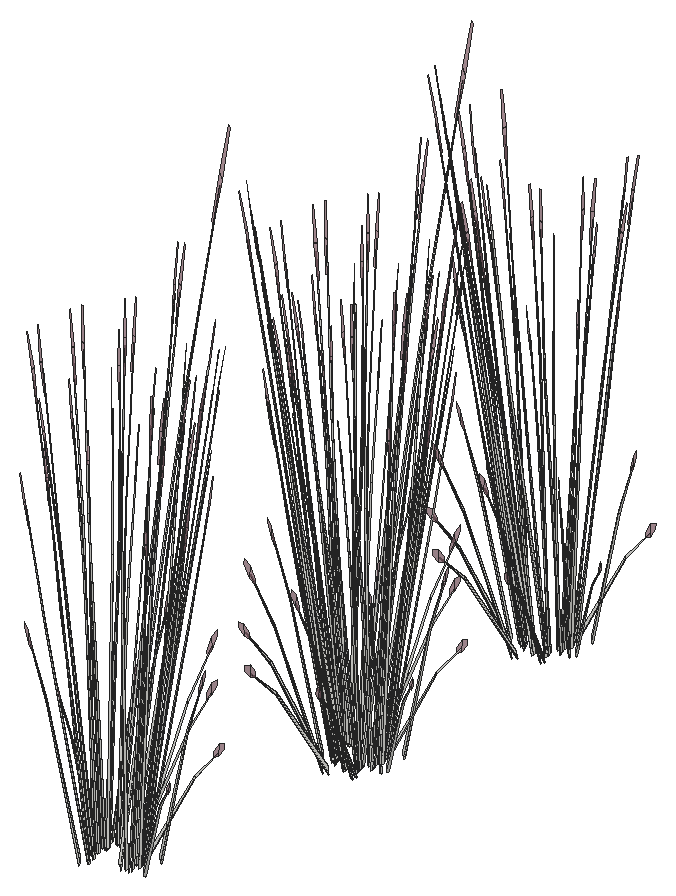
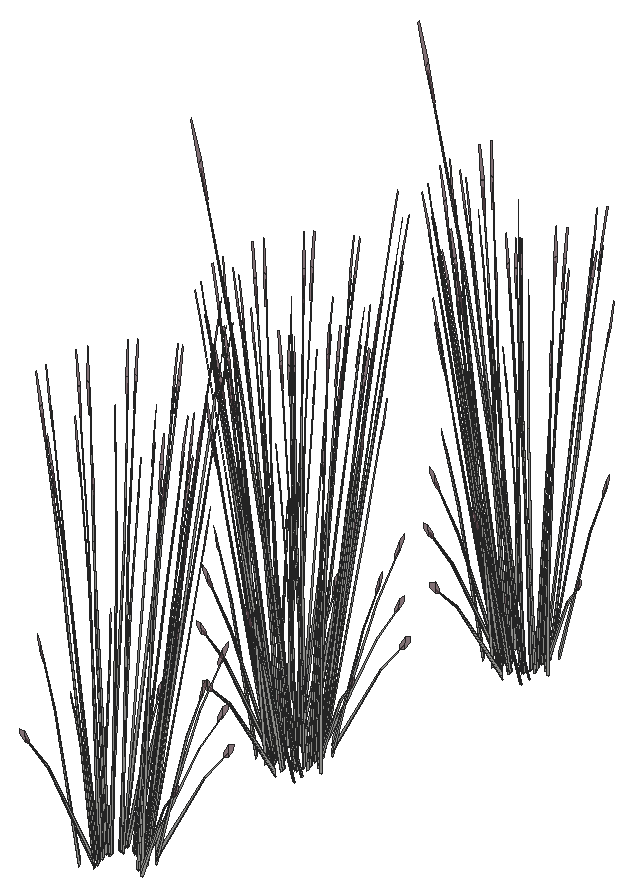
# SketchUp Ruby script. Lengths in inches.
U = 1.inch
M = Sketchup.active_model
def pt(a) = Geom::Point3d.new(a.map { |v| v * U })
def face(e, loops, mat)
  f = e.add_face(loops[0].map { |a| pt(a) })
  loops[1..].each { |l| e.add_face(l.map { |a| pt(a) }).erase! }
  f.material = f.back_material = mat if mat
  f
end
# faces: each face lists its corners as indices into pts; further lists are holes
def faces(e, pts, list, mat = nil) = list.each { |f| face(e, (f[0].is_a?(Array) ? f : [f]).map { |l| l.map { |i| pts[i] } }, mat) }
# xy, xz, yz: faces in a plane at the given z, y or x. An outline is a flat list of corners, or four numbers for a rectangle; further outlines are holes
def ring(l) = l.size == 4 ? [[l[0], l[1]], [l[2], l[1]], [l[2], l[3]], [l[0], l[3]]] : l.each_slice(2).to_a
def flat(e, list, mat, &to3) = list.each { |f| face(e, (f[0].is_a?(Array) ? f : [f]).map { |l| ring(l).map { |u, v| to3.(u, v) } }, mat) }
def xy(e, z, list, mat = nil) = flat(e, list, mat) { |x, y| [x, y, z] }
def xz(e, y, list, mat = nil) = flat(e, list, mat) { |x, z| [x, y, z] }
def yz(e, x, list, mat = nil) = flat(e, list, mat) { |y, z| [x, y, z] }
def lines(e, pts, list) = list.each { |a, b| e.add_line(pt(pts[a]), pt(pts[b])) }
# prism: a flat outline (further loops are holes) pulled along v
def prism(e, loops, v, mat = nil)
  f = face(e, loops, mat); d = Geom::Vector3d.new(v.map { |x| x * U })
  f.pushpull(f.normal.samedirection?(d) ? d.length : -d.length)
end
def box(e, o, s, mat = nil) = prism(e, [[o, [o[0] + s[0], o[1], o[2]], [o[0] + s[0], o[1] + s[1], o[2]], [o[0], o[1] + s[1], o[2]]]], [0, 0, s[2]], mat)
def at(x, y, z, deg = 0) = Geom::Transformation.translation(pt([x, y, z])) * Geom::Transformation.rotation(ORIGIN, Z_AXIS, deg.degrees)
def axes(o, x, y, z) = Geom::Transformation.new([*x, 0, *y, 0, *z, 0, *pt(o).to_a, 1])
def part(name) = M.definitions.add(name)
# library, detail: a bought-in or finely detailed component or shape, given as its bounding box
def library(name, o, s) = part(name).tap { |d| box(d.entities, o, s) }
def detail(e, o, s) = box(e.add_group.entities, o, s)
def put(e, d, t, mat = nil) = e.add_instance(d, t).tap { |i| i.material = mat if mat }
def group(e, t, mat = nil) = e.add_group.tap { |g| g.transformation = t; g.material = mat if mat }.entities
root = M.entities
M.materials.add("LightPink_Translucent").color = [144, 107, 117]
M.materials["LightPink_Translucent"].alpha = 0.75
c1 = part("blade")
p = [[2.15,0.21,22],[0,0.17,0],[0.09,0.45,0],[2.18,0.31,22],[2.29,0.31,22],[0.38,0.45,0],
  [2.48,0.24,33],[2.49,0.24,33],[2.48,0.22,33]]
faces(c1.entities,p,[[0,1,2,3],[4,5,2,3],[6,3,4,7],[8,0,3,6]])
c2 = part("seeds")
p = [[0.3,-0.1,1.38],[-0.01,-0.03,1.59],[-0.01,-0.03,0.03],[0.14,-0.07,-0.07],[0.29,-0.03,3],[0.15,0.01,3.11]]
faces(c2.entities,p,[[0,1,2,3],[1,0,4,5]],"LightPink_Translucent")
c3 = part("blade with seeds")
put(c3.entities,c1,at(0,0,0))
put(c3.entities,c2,axes([2.4,0.25,30.99],[1.5799,-0.05474,1.17369],[-0.12525,1.92788,0.29478],[-0.07173,-0.02425,1.56792]))
put(root,c3,axes([397.1875,39.03,4.73],[0.01777,-0.35463,0.0643],[0.26836,0.00972,0.50621],[-0.1028,-0.03711,0.77189]))
put(root,c3,axes([399.82,39.89,5.05],[-0.30722,0.06665,0.35414],[-0.08112,-0.381,-0.4572],[0.08804,-0.10234,0.87481]))
put(root,c3,axes([400.1,39.83,4.73],[0.2423,0.19613,0.0643],[-0.14107,0.2793,0.50621],[0.07768,-0.0903,0.77189]))
put(root,c3,axes([400.03,39.75,4.73],[0.08753,0.42921,0.48003],[-0.34336,0.07449,0.3958],[0.1012,-0.10094,0.9933]))
put(root,c3,axes([400.96,40.27,4.72],[0.04898,-0.07104,1.74944],[-0.06269,-0.43574,-0.27667],[0.12289,-0.08262,0.14031]))
put(root,c3,axes([396.82,38.57,4.71],[0.02617,0.04654,1.77383],[-0.12614,0.41836,-0.16761],[-0.12775,0.00303,0.31391]))
put(root,c3,axes([397.37,39.3,5.05],[0.20082,0.29199,0.35414],[-0.2293,0.2764,-0.4572],[-0.1165,-0.04206,0.87481]))
put(root,c3,axes([397.32,39.11,5.03],[-0.0189,0.47427,-0.1216],[-0.35781,-0.01296,-0.67495],[-0.13781,-0.03295,1.02557]))
put(root,c3,axes([399.99,40.93,5.03],[-0.17758,-0.42229,-0.1216],[0.31518,-0.20752,-0.67495],[0.13282,-0.05572,1.02557]))
put(root,c3,axes([399.87,40.81,5.05],[-0.29332,-0.1301,0.35414],[0.08555,-0.37955,-0.4572],[0.11809,-0.0348,0.87481]))
put(root,c3,axes([396.8,40.11,4.73],[0.09971,-0.42522,0.48003],[0.32782,0.1454,0.3958],[-0.12892,0.02555,0.9933]))
put(root,c3,axes([396.77,40,4.73],[-0.12963,-0.31798,0.0643],[0.23638,-0.15564,0.50621],[-0.1042,0.03071,0.77189]))
put(root,c3,axes([400.14,40.92,4.73],[0.12963,0.31798,0.0643],[-0.23638,0.15564,0.50621],[0.1042,-0.03071,0.77189]))
put(root,c3,axes([400.11,40.81,4.73],[-0.09971,0.42522,0.48003],[-0.32782,-0.1454,0.3958],[0.12892,-0.02555,0.9933]))
put(root,c3,axes([397.04,40.12,5.05],[0.29332,0.1301,0.35414],[-0.08555,0.37955,-0.4572],[-0.11809,0.0348,0.87481]))
put(root,c3,axes([400.7,42.1875,4.71],[-0.03191,-0.04083,1.77383],[0.06981,-0.43764,-0.16761],[0.12571,-0.02796,0.31391]))
put(root,c3,axes([396.55,40.41,4.72],[-0.05763,0.06055,1.74944],[0.0049,0.44239,-0.27667],[-0.13211,0.05753,0.14031]))
put(root,c3,axes([396.92,39.99,5.03],[0.17758,0.42229,-0.1216],[-0.31518,0.20752,-0.67495],[-0.13282,0.05572,1.02557]))
put(root,c3,axes([399.59,41.81,5.03],[0.0189,-0.47427,-0.1216],[0.35781,0.01296,-0.67495],[0.13781,0.03295,1.02557]))
put(root,c3,axes([399.54,41.625,5.05],[-0.20082,-0.29199,0.35414],[0.2293,-0.2764,-0.4572],[0.1165,0.04206,0.87481]))
put(root,c3,axes([399.91,41.53,4.72],[0.07571,-0.00789,1.74944],[0.20767,-0.36231,-0.27667],[0.13467,0.04783,0.14031]))
put(root,c3,axes([396.88,41.17,4.73],[-0.08753,-0.42921,0.48003],[0.34336,-0.07449,0.3958],[-0.1012,0.10094,0.9933]))
put(root,c3,axes([396.81,41.09,4.73],[-0.2423,-0.19613,0.0643],[0.14107,-0.2793,0.50621],[-0.07768,0.0903,0.77189]))
put(root,c3,axes([397.09,41.03,5.05],[0.30722,-0.06665,0.35414],[0.08112,0.381,-0.4572],[-0.08804,0.10234,0.87481]))
put(root,c3,axes([395.91,40.86,4.71],[0.04504,0.01251,1.77383],[0.13934,0.41205,-0.16761],[-0.0922,0.10815,0.31391]))
put(root,c3,axes([399.72,41.89,4.73],[-0.01777,0.35463,0.0643],[-0.26836,-0.00972,0.50621],[0.1028,0.03711,0.77189]))
put(root,c3,axes([399.75,41.78,4.73],[-0.26024,0.30729,0.48003],[-0.22444,-0.32634,0.3958],[0.1221,0.05668,0.9933]))
put(root,c3,axes([396.39,42.11,5.65],[0.31145,0.12449,-0.06488],[-0.0958,0.38314,-0.29416],[-0.05094,0.05817,0.97024]))
put(root,c3,axes([398.92,42.13,5.05],[-0.05451,-0.37564,0.35414],[0.31161,-0.09919,-0.4572],[0.0837,0.10765,0.87481]))
put(root,c3,axes([399.13,39.97,4.47],[-0.30498,-0.24231,1.38283],[0.32203,-0.37727,0.59665],[0.0984,0.22736,1.33663]))
put(root,c3,axes([396.93,40.99,5.03],[0.32648,0.25715,-0.1216],[-0.18809,0.3724,-0.67495],[-0.09224,0.12945,1.02557]))
put(root,c3,axes([398.89,42.33,5.03],[0.21031,-0.39918,-0.1216],[0.30457,0.22997,-0.67495],[0.10587,0.11278,1.02557]))
put(root,c3,axes([397.5,41.79,5.05],[0.23881,-0.24554,0.35414],[0.22606,0.28036,-0.4572],[-0.0344,0.14245,0.87481]))
put(root,c3,axes([398.61,42.66,4.71],[0.00104,-0.05646,1.77383],[0.30246,-0.2491,-0.16761],[0.10506,0.08891,0.31391]))
put(root,c3,axes([397.29,42.01,4.73],[-0.29004,-0.02173,0.0643],[0.00795,-0.32812,0.50621],[-0.03035,0.12569,0.77189]))
put(root,c3,axes([397.38,42.04,4.73],[-0.25132,-0.3182,0.48003],[0.2669,-0.27442,0.3958],[-0.04636,0.14929,0.9933]))
put(root,c3,axes([398.17,42.19,5.05],[0.1064,-0.35863,0.35414],[0.31043,0.1046,-0.4572],[0.02846,0.14439,0.87481]))
put(root,c3,axes([398.97,42.47,4.73],[-0.16041,0.29625,0.0643],[-0.22843,-0.17248,0.50621],[0.07385,0.09498,0.77189]))
put(root,c3,axes([398.59,43.47,5.65],[0.2439,-0.26754,-0.06488],[0.22348,0.29302,-0.29416],[0.01573,0.08303,0.97024]))
put(root,c3,axes([399.04,42.39,4.73],[-0.35104,0.10702,0.48003],[-0.06092,-0.41983,0.3958],[0.08256,0.12373,0.9933]))
put(root,c3,axes([398.08,42.52,4.73],[-0.26007,0.1585,0.0643],[-0.12729,-0.28902,0.50621],[0.02512,0.1274,0.77189]))
put(root,c3,axes([396.56,42.0625,4.72],[-0.00877,0.09229,1.74944],[0.24897,0.32105,-0.27667],[-0.06518,0.15182,0.14031]))
put(root,c3,axes([397.35,41.85,5.4],[0.3879,0.02311,-0.13498],[-0.0106,0.43749,-0.74919],[-0.02694,0.1685,1.13838]))
put(root,c3,axes([398.07,42.34,5.03],[0.34538,-0.21713,-0.1216],[0.16972,0.38536,-0.67495],[0.04557,0.16239,1.02557]))
put(root,c3,axes([398.17,42.49,5.0625],[-0.34777,-0.12192,0.53283],[0.11892,-0.40083,0.43934],[0.0209,0.15763,1.10256]))
put(root,c3,axes([396.53,43.01,4.71],[0.04004,-0.02816,1.77383],[0.33095,0.18728,-0.16761],[-0.00778,0.15594,0.31391]))
put(root,c3,axes([397.99,43.2,4.72],[0.04474,0.0751,1.74944],[0.36104,0.0295,-0.27667],[0.03631,0.16562,0.14031]))
put(root,c3,axes([401.89,57.67,4.72],[-0.05398,-0.06539,1.74944],[-0.36026,0.04145,-0.27667],[-0.0575,-0.15639,0.14031]))
put(root,c3,axes([403.51,58.47,4.72],[-0.00341,-0.09282,1.74944],[-0.28775,-0.26825,-0.27667],[0.04449,-0.16261,0.14031]))
put(root,c3,axes([403.43,58.13,4.71],[-0.03584,0.03562,1.77383],[-0.35118,-0.12018,-0.16761],[-0.01271,-0.15545,0.31391]))
put(root,c3,axes([401.52,57.45,4.71],[-0.00658,0.0559,1.77383],[-0.32474,0.20287,-0.16761],[-0.09556,-0.1037,0.31391]))
put(root,c3,axes([401.45,58.44,5.09],[0.39316,-0.11987,0.53763],[0.06823,0.47021,0.4433],[-0.09247,-0.13858,1.11249]))
put(root,c3,axes([402.34,58.53,4.73],[0.34777,0.12192,0.48003],[-0.11892,0.40083,0.3958],[-0.0209,-0.15763,0.9933]))
put(root,c3,axes([402.4375,58.68,5.03],[-0.34538,0.21713,-0.1216],[-0.16972,-0.38536,-0.67495],[-0.04557,-0.16239,1.02557]))
put(root,c3,axes([403.15,59.16,5.03],[-0.3879,-0.02311,-0.1216],[0.0106,-0.43749,-0.67495],[0.02694,-0.1685,1.02557]))
put(root,c3,axes([402.43,58.5,4.73],[0.26007,-0.1585,0.0643],[0.12729,0.28902,0.50621],[-0.02512,-0.1274,0.77189]))
put(root,c3,axes([401.54,58.55,4.73],[0.16041,-0.29625,0.0643],[0.22843,0.17248,0.50621],[-0.07385,-0.09498,0.77189]))
put(root,c3,axes([402.33,58.83,5.05],[-0.1064,0.35863,0.35414],[-0.31043,-0.1046,-0.4572],[-0.02846,-0.14439,0.87481]))
put(root,c3,axes([403.125,58.98,4.73],[0.25132,0.3182,0.48003],[-0.2669,0.27442,0.3958],[0.04636,-0.14929,0.9933]))
put(root,c3,axes([401.61,58.52,5.43],[-0.23555,0.44708,-0.13619],[-0.34112,-0.25757,-0.75594],[-0.11858,-0.12631,1.14864]))
put(root,c3,axes([403.22,59.01,4.73],[0.29004,0.02173,0.0643],[-0.00795,0.32812,0.50621],[0.03035,-0.12569,0.77189]))
put(root,c3,axes([403,59.23,5.05],[-0.23881,0.24554,0.35414],[-0.22606,-0.28036,-0.4572],[0.0344,-0.14245,0.87481]))
put(root,c3,axes([400.71,58.39,4.72],[-0.07594,-0.00329,1.74944],[-0.24177,0.32918,-0.27667],[-0.129,-0.06726,0.14031]))
put(root,c3,axes([403.58,60.02,5.03],[-0.32648,-0.25715,-0.1216],[0.18809,-0.3724,-0.67495],[0.09224,-0.12945,1.02557]))
put(root,c3,axes([401.59,58.89,5.05],[0.05451,0.37564,0.35414],[-0.31161,0.09919,-0.4572],[-0.0837,-0.10765,0.87481]))
put(root,c3,axes([400.65,59.13,5.09],[0.29147,-0.34417,0.53763],[0.25138,0.3655,0.4433],[-0.13675,-0.06349,1.11249]))
put(root,c3,axes([404.38,59.91,4.71],[-0.0461,-0.00354,1.77383],[-0.19143,-0.37951,-0.16761],[0.07688,-0.12478,0.31391]))
put(root,c3,axes([400.78,59.13,4.73],[0.01777,-0.35463,0.0643],[0.26836,0.00972,0.50621],[-0.1028,-0.03711,0.77189]))
put(root,c3,axes([403.42,59.99,5.05],[-0.30722,0.06665,0.35414],[-0.08112,-0.381,-0.4572],[0.08804,-0.10234,0.87481]))
put(root,c3,axes([403.7,59.93,4.73],[0.2423,0.19613,0.0643],[-0.14107,0.2793,0.50621],[0.07768,-0.0903,0.77189]))
put(root,c3,axes([403.63,59.85,4.73],[0.08753,0.42921,0.48003],[-0.34336,0.07449,0.3958],[0.1012,-0.10094,0.9933]))
put(root,c3,axes([404.55,60.37,4.72],[0.04898,-0.07104,1.74944],[-0.06269,-0.43574,-0.27667],[0.12289,-0.08262,0.14031]))
put(root,c3,axes([400.42,58.67,4.71],[0.02617,0.04654,1.77383],[-0.12614,0.41836,-0.16761],[-0.12775,0.00303,0.31391]))
put(root,c3,axes([400.97,59.39,5.05],[0.20082,0.29199,0.35414],[-0.2293,0.2764,-0.4572],[-0.1165,-0.04206,0.87481]))
put(root,c3,axes([400.91,59.21,5.03],[-0.0189,0.47427,-0.1216],[-0.35781,-0.01296,-0.67495],[-0.13781,-0.03295,1.02557]))
put(root,c3,axes([403.59,61.03,5.03],[-0.17758,-0.42229,-0.1216],[0.31518,-0.20752,-0.67495],[0.13282,-0.05572,1.02557]))
put(root,c3,axes([403.47,60.9,5.05],[-0.29332,-0.1301,0.35414],[0.08555,-0.37955,-0.4572],[0.11809,-0.0348,0.87481]))
put(root,c3,axes([400.4,60.21,4.73],[0.09971,-0.42522,0.48003],[0.32782,0.1454,0.3958],[-0.12892,0.02555,0.9933]))
put(root,c3,axes([400.37,60.09,4.73],[-0.12963,-0.31798,0.0643],[0.23638,-0.15564,0.50621],[-0.1042,0.03071,0.77189]))
put(root,c3,axes([403.73,61.02,4.73],[0.12963,0.31798,0.0643],[-0.23638,0.15564,0.50621],[0.1042,-0.03071,0.77189]))
put(root,c3,axes([403.71,60.91,4.73],[-0.09971,0.42522,0.48003],[-0.32782,-0.1454,0.3958],[0.12892,-0.02555,0.9933]))
put(root,c3,axes([400.64,60.21,5.05],[0.29332,0.1301,0.35414],[-0.08555,0.37955,-0.4572],[-0.11809,0.0348,0.87481]))
put(root,c3,axes([404.3,62.28,4.71],[-0.03191,-0.04083,1.77383],[0.06981,-0.43764,-0.16761],[0.12571,-0.02796,0.31391]))
put(root,c3,axes([400.14,60.51,4.72],[-0.05763,0.06055,1.74944],[0.0049,0.44239,-0.27667],[-0.13211,0.05753,0.14031]))
put(root,c3,axes([400.51,60.09,5.03],[0.17758,0.42229,-0.1216],[-0.31518,0.20752,-0.67495],[-0.13282,0.05572,1.02557]))
put(root,c3,axes([403.19,61.91,5.03],[0.0189,-0.47427,-0.1216],[0.35781,0.01296,-0.67495],[0.13781,0.03295,1.02557]))
put(root,c3,axes([403.14,61.72,5.05],[-0.20082,-0.29199,0.35414],[0.2293,-0.2764,-0.4572],[0.1165,0.04206,0.87481]))
put(root,c3,axes([403.5,61.62,4.72],[0.07571,-0.00789,1.74944],[0.20767,-0.36231,-0.27667],[0.13467,0.04783,0.14031]))
put(root,c3,axes([400.47,61.27,4.73],[-0.08753,-0.42921,0.48003],[0.34336,-0.07449,0.3958],[-0.1012,0.10094,0.9933]))
put(root,c3,axes([400.41,61.18,4.73],[-0.2423,-0.19613,0.0643],[0.14107,-0.2793,0.50621],[-0.07768,0.0903,0.77189]))
put(root,c3,axes([400.6875,61.125,5.05],[0.30722,-0.06665,0.35414],[0.08112,0.381,-0.4572],[-0.08804,0.10234,0.87481]))
put(root,c3,axes([399.5,60.95,4.71],[0.04504,0.01251,1.77383],[0.13934,0.41205,-0.16761],[-0.0922,0.10815,0.31391]))
put(root,c3,axes([403.32,61.98,4.73],[-0.01777,0.35463,0.0643],[-0.26836,-0.00972,0.50621],[0.1028,0.03711,0.77189]))
put(root,c3,axes([403.34,61.87,4.73],[-0.26024,0.30729,0.48003],[-0.22444,-0.32634,0.3958],[0.1221,0.05668,0.9933]))
put(root,c3,axes([399.99,62.21,5.65],[0.31145,0.12449,-0.06488],[-0.0958,0.38314,-0.29416],[-0.05094,0.05817,0.97024]))
put(root,c3,axes([402.52,62.23,5.05],[-0.05451,-0.37564,0.35414],[0.31161,-0.09919,-0.4572],[0.0837,0.10765,0.87481]))
put(root,c3,axes([402.72,60.07,4.47],[-0.30498,-0.24231,1.38283],[0.32203,-0.37727,0.59665],[0.0984,0.22736,1.33663]))
put(root,c3,axes([400.53,61.09,5.03],[0.32648,0.25715,-0.1216],[-0.18809,0.3724,-0.67495],[-0.09224,0.12945,1.02557]))
put(root,c3,axes([402.49,62.42,5.03],[0.21031,-0.39918,-0.1216],[0.30457,0.22997,-0.67495],[0.10587,0.11278,1.02557]))
put(root,c3,axes([401.1,61.88,5.05],[0.23881,-0.24554,0.35414],[0.22606,0.28036,-0.4572],[-0.0344,0.14245,0.87481]))
put(root,c3,axes([402.21,62.75,4.71],[0.00104,-0.05646,1.77383],[0.30246,-0.2491,-0.16761],[0.10506,0.08891,0.31391]))
put(root,c3,axes([400.88,62.11,4.73],[-0.29004,-0.02173,0.0643],[0.00795,-0.32812,0.50621],[-0.03035,0.12569,0.77189]))
put(root,c3,axes([400.98,62.14,4.73],[-0.25132,-0.3182,0.48003],[0.2669,-0.27442,0.3958],[-0.04636,0.14929,0.9933]))
put(root,c3,axes([401.77,62.29,5.05],[0.1064,-0.35863,0.35414],[0.31043,0.1046,-0.4572],[0.02846,0.14439,0.87481]))
put(root,c3,axes([402.56,62.57,4.73],[-0.16041,0.29625,0.0643],[-0.22843,-0.17248,0.50621],[0.07385,0.09498,0.77189]))
put(root,c3,axes([402.1875,63.57,5.65],[0.2439,-0.26754,-0.06488],[0.22348,0.29302,-0.29416],[0.01573,0.08303,0.97024]))
put(root,c3,axes([402.63,62.48,4.73],[-0.35104,0.10702,0.48003],[-0.06092,-0.41983,0.3958],[0.08256,0.12373,0.9933]))
put(root,c3,axes([401.67,62.61,4.73],[-0.26007,0.1585,0.0643],[-0.12729,-0.28902,0.50621],[0.02512,0.1274,0.77189]))
put(root,c3,axes([400.15,62.16,4.72],[-0.00877,0.09229,1.74944],[0.24897,0.32105,-0.27667],[-0.06518,0.15182,0.14031]))
put(root,c3,axes([400.95,61.95,5.4],[0.3879,0.02311,-0.13498],[-0.0106,0.43749,-0.74919],[-0.02694,0.1685,1.13838]))
put(root,c3,axes([401.67,62.4375,5.03],[0.34538,-0.21713,-0.1216],[0.16972,0.38536,-0.67495],[0.04557,0.16239,1.02557]))
put(root,c3,axes([401.77,62.58,5.0625],[-0.34777,-0.12192,0.53283],[0.11892,-0.40083,0.43934],[0.0209,0.15763,1.10256]))
put(root,c3,axes([400.125,63.1,4.71],[0.04004,-0.02816,1.77383],[0.33095,0.18728,-0.16761],[-0.00778,0.15594,0.31391]))
put(root,c3,axes([401.58,63.3,4.72],[0.04474,0.0751,1.74944],[0.36104,0.0295,-0.27667],[0.03631,0.16562,0.14031]))
put(root,c3,axes([401.89,76.76,4.72],[-0.05398,-0.06539,1.74944],[-0.36026,0.04145,-0.27667],[-0.0575,-0.15639,0.14031]))
put(root,c3,axes([403.51,77.5625,4.72],[-0.00341,-0.09282,1.74944],[-0.28775,-0.26825,-0.27667],[0.04449,-0.16261,0.14031]))
put(root,c3,axes([403.43,77.23,4.71],[-0.03584,0.03562,1.77383],[-0.35118,-0.12018,-0.16761],[-0.01271,-0.15545,0.31391]))
put(root,c3,axes([401.52,76.55,4.71],[-0.00658,0.0559,1.77383],[-0.32474,0.20287,-0.16761],[-0.09556,-0.1037,0.31391]))
put(root,c3,axes([401.45,77.54,5.09],[0.39316,-0.11987,0.53763],[0.06823,0.47021,0.4433],[-0.09247,-0.13858,1.11249]))
put(root,c3,axes([402.34,77.63,4.73],[0.34777,0.12192,0.48003],[-0.11892,0.40083,0.3958],[-0.0209,-0.15763,0.9933]))
put(root,c3,axes([402.4375,77.77,5.03],[-0.34538,0.21713,-0.1216],[-0.16972,-0.38536,-0.67495],[-0.04557,-0.16239,1.02557]))
put(root,c3,axes([403.15,78.26,5.03],[-0.3879,-0.02311,-0.1216],[0.0106,-0.43749,-0.67495],[0.02694,-0.1685,1.02557]))
put(root,c3,axes([402.43,77.6,4.73],[0.26007,-0.1585,0.0643],[0.12729,0.28902,0.50621],[-0.02512,-0.1274,0.77189]))
put(root,c3,axes([401.54,77.64,4.73],[0.16041,-0.29625,0.0643],[0.22843,0.17248,0.50621],[-0.07385,-0.09498,0.77189]))
put(root,c3,axes([402.33,77.92,5.05],[-0.1064,0.35863,0.35414],[-0.31043,-0.1046,-0.4572],[-0.02846,-0.14439,0.87481]))
put(root,c3,axes([403.125,78.07,4.73],[0.25132,0.3182,0.48003],[-0.2669,0.27442,0.3958],[0.04636,-0.14929,0.9933]))
put(root,c3,axes([401.61,77.61,5.43],[-0.23555,0.44708,-0.13619],[-0.34112,-0.25757,-0.75594],[-0.11858,-0.12631,1.14864]))
put(root,c3,axes([403.22,78.1,4.73],[0.29004,0.02173,0.0643],[-0.00795,0.32812,0.50621],[0.03035,-0.12569,0.77189]))
put(root,c3,axes([403,78.33,5.05],[-0.23881,0.24554,0.35414],[-0.22606,-0.28036,-0.4572],[0.0344,-0.14245,0.87481]))
put(root,c3,axes([400.71,77.48,4.72],[-0.07594,-0.00329,1.74944],[-0.24177,0.32918,-0.27667],[-0.129,-0.06726,0.14031]))
put(root,c3,axes([403.58,79.12,5.03],[-0.32648,-0.25715,-0.1216],[0.18809,-0.3724,-0.67495],[0.09224,-0.12945,1.02557]))
put(root,c3,axes([401.59,77.98,5.05],[0.05451,0.37564,0.35414],[-0.31161,0.09919,-0.4572],[-0.0837,-0.10765,0.87481]))
put(root,c3,axes([400.65,78.23,5.09],[0.29147,-0.34417,0.53763],[0.25138,0.3655,0.4433],[-0.13675,-0.06349,1.11249]))
put(root,c3,axes([404.38,79.01,4.71],[-0.0461,-0.00354,1.77383],[-0.19143,-0.37951,-0.16761],[0.07688,-0.12478,0.31391]))
put(root,c3,axes([400.78,78.22,4.73],[0.01777,-0.35463,0.0643],[0.26836,0.00972,0.50621],[-0.1028,-0.03711,0.77189]))
put(root,c3,axes([403.42,79.09,5.05],[-0.30722,0.06665,0.35414],[-0.08112,-0.381,-0.4572],[0.08804,-0.10234,0.87481]))
put(root,c3,axes([403.7,79.03,4.73],[0.2423,0.19613,0.0643],[-0.14107,0.2793,0.50621],[0.07768,-0.0903,0.77189]))
put(root,c3,axes([403.63,78.94,4.73],[0.08753,0.42921,0.48003],[-0.34336,0.07449,0.3958],[0.1012,-0.10094,0.9933]))
put(root,c3,axes([404.55,79.46,4.72],[0.04898,-0.07104,1.74944],[-0.06269,-0.43574,-0.27667],[0.12289,-0.08262,0.14031]))
put(root,c3,axes([400.42,77.76,4.71],[0.02617,0.04654,1.77383],[-0.12614,0.41836,-0.16761],[-0.12775,0.00303,0.31391]))
put(root,c3,axes([400.97,78.49,5.05],[0.20082,0.29199,0.35414],[-0.2293,0.2764,-0.4572],[-0.1165,-0.04206,0.87481]))
put(root,c3,axes([400.91,78.3,5.03],[-0.0189,0.47427,-0.1216],[-0.35781,-0.01296,-0.67495],[-0.13781,-0.03295,1.02557]))
put(root,c3,axes([403.59,80.125,5.03],[-0.17758,-0.42229,-0.1216],[0.31518,-0.20752,-0.67495],[0.13282,-0.05572,1.02557]))
put(root,c3,axes([403.47,80,5.05],[-0.29332,-0.1301,0.35414],[0.08555,-0.37955,-0.4572],[0.11809,-0.0348,0.87481]))
put(root,c3,axes([400.4,79.3,4.73],[0.09971,-0.42522,0.48003],[0.32782,0.1454,0.3958],[-0.12892,0.02555,0.9933]))
put(root,c3,axes([400.37,79.19,4.73],[-0.12963,-0.31798,0.0643],[0.23638,-0.15564,0.50621],[-0.1042,0.03071,0.77189]))
put(root,c3,axes([403.73,80.11,4.73],[0.12963,0.31798,0.0643],[-0.23638,0.15564,0.50621],[0.1042,-0.03071,0.77189]))
put(root,c3,axes([403.71,80,4.73],[-0.09971,0.42522,0.48003],[-0.32782,-0.1454,0.3958],[0.12892,-0.02555,0.9933]))
put(root,c3,axes([400.64,79.31,5.05],[0.29332,0.1301,0.35414],[-0.08555,0.37955,-0.4572],[-0.11809,0.0348,0.87481]))
put(root,c3,axes([404.3,81.38,4.71],[-0.03191,-0.04083,1.77383],[0.06981,-0.43764,-0.16761],[0.12571,-0.02796,0.31391]))
put(root,c3,axes([400.14,79.6,4.72],[-0.05763,0.06055,1.74944],[0.0049,0.44239,-0.27667],[-0.13211,0.05753,0.14031]))
put(root,c3,axes([400.51,79.18,5.03],[0.17758,0.42229,-0.1216],[-0.31518,0.20752,-0.67495],[-0.13282,0.05572,1.02557]))
put(root,c3,axes([403.19,81,5.03],[0.0189,-0.47427,-0.1216],[0.35781,0.01296,-0.67495],[0.13781,0.03295,1.02557]))
put(root,c3,axes([403.14,80.82,5.05],[-0.20082,-0.29199,0.35414],[0.2293,-0.2764,-0.4572],[0.1165,0.04206,0.87481]))
put(root,c3,axes([403.5,80.72,4.72],[0.07571,-0.00789,1.74944],[0.20767,-0.36231,-0.27667],[0.13467,0.04783,0.14031]))
